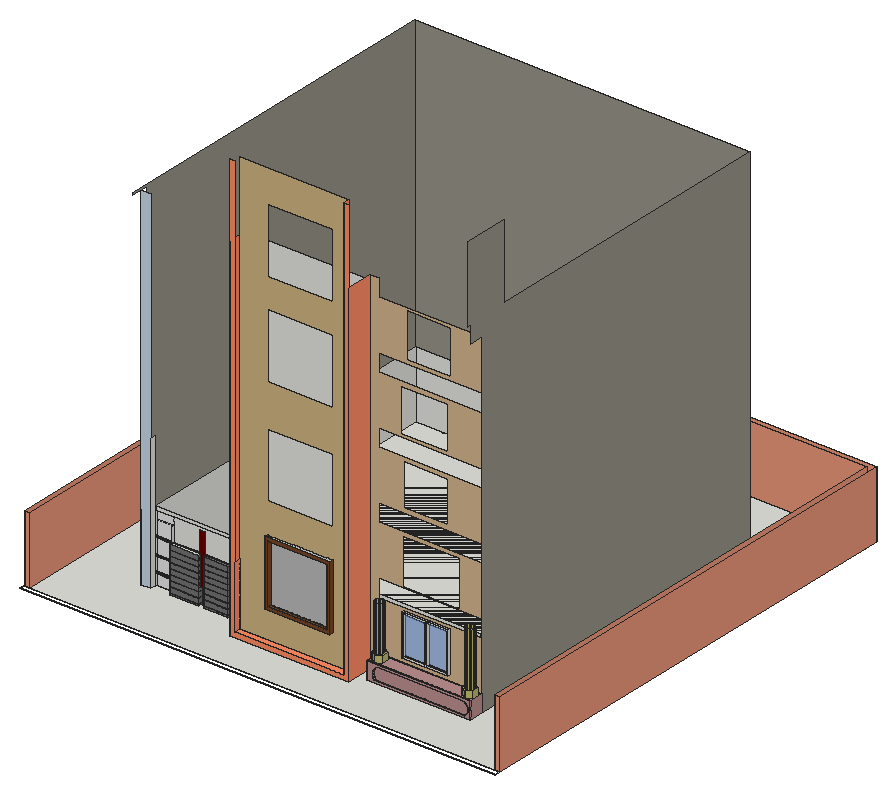
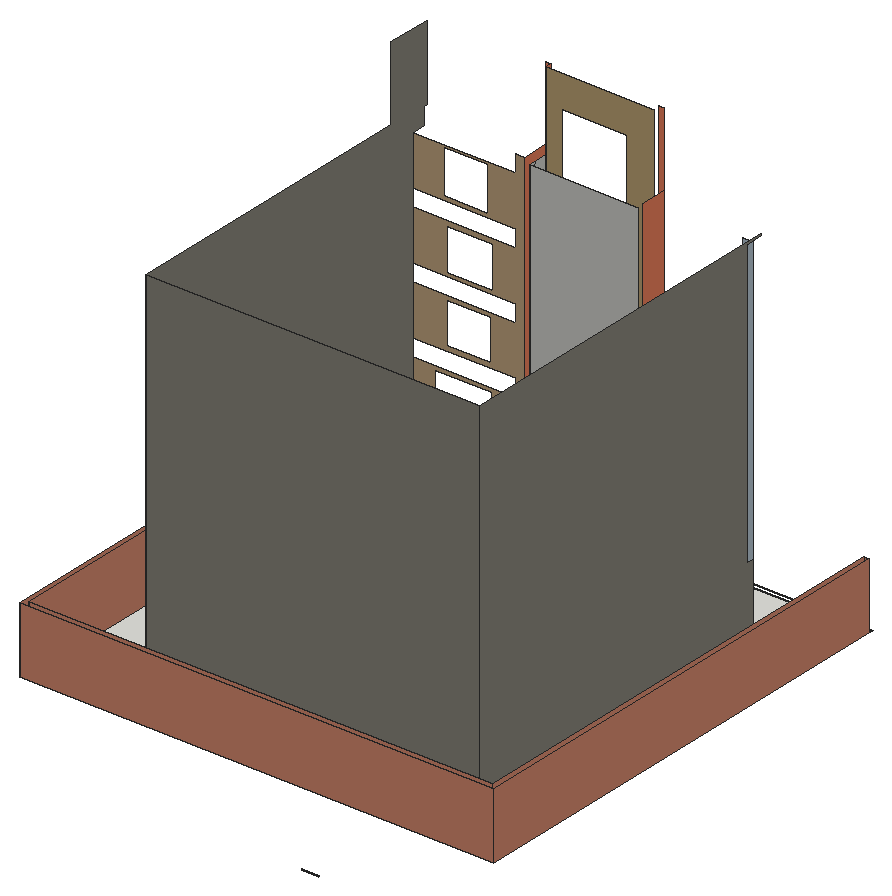
# SketchUp Ruby script. Lengths in inches.
U = 1.inch
M = Sketchup.active_model
def pt(a) = Geom::Point3d.new(a.map { |v| v * U })
def face(e, loops, mat)
  f = e.add_face(loops[0].map { |a| pt(a) })
  loops[1..].each { |l| e.add_face(l.map { |a| pt(a) }).erase! }
  f.material = f.back_material = mat if mat
  f
end
# faces: each face lists its corners as indices into pts; further lists are holes
def faces(e, pts, list, mat = nil) = list.each { |f| face(e, (f[0].is_a?(Array) ? f : [f]).map { |l| l.map { |i| pts[i] } }, mat) }
# xy, xz, yz: faces in a plane at the given z, y or x. An outline is a flat list of corners, or four numbers for a rectangle; further outlines are holes
def ring(l) = l.size == 4 ? [[l[0], l[1]], [l[2], l[1]], [l[2], l[3]], [l[0], l[3]]] : l.each_slice(2).to_a
def flat(e, list, mat, &to3) = list.each { |f| face(e, (f[0].is_a?(Array) ? f : [f]).map { |l| ring(l).map { |u, v| to3.(u, v) } }, mat) }
def xy(e, z, list, mat = nil) = flat(e, list, mat) { |x, y| [x, y, z] }
def xz(e, y, list, mat = nil) = flat(e, list, mat) { |x, z| [x, y, z] }
def yz(e, x, list, mat = nil) = flat(e, list, mat) { |y, z| [x, y, z] }
def lines(e, pts, list) = list.each { |a, b| e.add_line(pt(pts[a]), pt(pts[b])) }
# prism: a flat outline (further loops are holes) pulled along v
def prism(e, loops, v, mat = nil)
  f = face(e, loops, mat); d = Geom::Vector3d.new(v.map { |x| x * U })
  f.pushpull(f.normal.samedirection?(d) ? d.length : -d.length)
end
def box(e, o, s, mat = nil) = prism(e, [[o, [o[0] + s[0], o[1], o[2]], [o[0] + s[0], o[1] + s[1], o[2]], [o[0], o[1] + s[1], o[2]]]], [0, 0, s[2]], mat)
def at(x, y, z, deg = 0) = Geom::Transformation.translation(pt([x, y, z])) * Geom::Transformation.rotation(ORIGIN, Z_AXIS, deg.degrees)
def axes(o, x, y, z) = Geom::Transformation.new([*x, 0, *y, 0, *z, 0, *pt(o).to_a, 1])
def part(name) = M.definitions.add(name)
# library, detail: a bought-in or finely detailed component or shape, given as its bounding box
def library(name, o, s) = part(name).tap { |d| box(d.entities, o, s) }
def detail(e, o, s) = box(e.add_group.entities, o, s)
def put(e, d, t, mat = nil) = e.add_instance(d, t).tap { |i| i.material = mat if mat }
def group(e, t, mat = nil) = e.add_group.tap { |g| g.transformation = t; g.material = mat if mat }.entities
root = M.entities
M.materials.add("[0014_DarkSalmon]").color = [233, 150, 122]
M.materials.add("[0035_Tan]").color = [210, 180, 140]
M.materials.add("[0057_DarkKhaki]").color = [189, 183, 107]
M.materials.add("[0119_RosyBrown]").color = [188, 143, 143]
M.materials.add("[Color A08]").color = [102, 0, 0]
M.materials.add("[Color B03]").color = [255, 140, 101]
M.materials.add("[Color M05]").color = [114, 114, 114]
M.materials.add("[Color M09]").color = [0, 0, 0]
M.materials.add("[Formica Graystone]").color = [149, 146, 135]
M.materials.add("[Mirror 01]").color = [185, 185, 185]
M.materials.add("[Mirror 02]").color = [229, 229, 229]
M.materials.add("[Stone Sandstone Ashlar Light]").color = [206, 178, 128]
M.materials.add("[Terrazzo Light Blue]").color = [196, 214, 227]
M.materials.add("[Translucent Glass Blue]").color = [100, 149, 237]
M.materials["[Translucent Glass Blue]"].alpha = 0.5
M.materials.add("[Wood Veneer 01]").color = [120, 70, 37]
xy(root,0,[[0,0,0,841.73,850.73,841.73,850.73,0,841.73,0,841.73,832.73,9,832.73,9,0],[[9,0,841.73,832.73],[312.71,68.37,525.05,104.37],[540.59,89.37,725.37,92.37],[173.97,107.37,226.48,113.37],[235.11,107.37,278.99,113.37],[309.83,113.37,312.71,116.37],[142.36,113.37,143.68,116.37]],[[312.71,68.37,312.71,113.37,309.83,113.37,309.83,116.37,278.99,116.37,278.99,107.37,235.11,107.37,235.11,113.37,226.48,113.37,226.48,107.37,173.97,107.37,173.97,116.37,143.68,116.37,143.68,113.37,142.36,113.37,142.36,104.37,125.37,104.37,125.37,716.37,725.37,716.37,725.37,89.37,540.59,89.37,540.59,116.37,525.05,116.37,525.05,68.37],[0,-9,850.73,0]],[312.71,68.37,525.05,104.37],[540.59,89.37,725.37,92.37],
  [540.59,92.37,725.37,116.37],[[125.37,104.37,125.37,716.37,725.37,716.37,725.37,116.37,525.05,116.37,525.05,104.37,312.71,104.37,312.71,116.37,142.36,116.37,142.36,104.37],[134.37,125.37,716.37,707.37]],[173.97,107.37,183.17,113.37],[183.17,107.37,226.48,113.37],[235.11,107.37,278.99,113.37],
  [142.36,113.37,143.68,116.37],[173.97,113.37,278.99,116.37],[309.83,113.37,312.71,116.37],[134.37,125.37,716.37,707.37]])
xy(root,2.25,[[173.97,107.37,226.48,113.37]])
xy(root,3,[[555.14,89.37,714.79,92.37]],"[0119_RosyBrown]")
xy(root,3,[[235.11,107.37,278.99,113.37]],"[Color M05]")
xy(root,3.25,[[173.97,107.37,183.17,113.37],[183.17,107.37,226.48,113.37]])
xy(root,3.9375,[[235.11,107.37,278.99,113.37]])
xy(root,9,[[321.71,80.37,516.05,104.37],[321.71,104.37,516.05,116.37]])
xy(root,9,[[321.71,68.37,516.05,80.37]],"[Color B03]")
xy(root,12.0625,[[173.97,107.37,226.48,113.37]])
xy(root,12.75,[[235.11,107.37,278.99,113.37]],"[Color M05]")
xy(root,13.0625,[[173.97,107.37,183.17,113.37],[183.17,107.37,226.48,113.37]])
xy(root,13.6875,[[235.11,107.37,278.99,113.37]])
xy(root,21.05,[[143.99,113.37,173.97,116.37],[278.99,113.37,309.83,116.37]],"[Color M09]")
xy(root,21.875,[[173.97,107.37,226.48,113.37]])
xy(root,22.5,[[235.11,107.37,278.99,113.37]],"[Color M05]")
xy(root,22.62,[[143.99,113.37,173.97,116.37],[278.99,113.37,309.83,116.37]],"[Color M09]")
xy(root,22.875,[[173.97,107.37,183.17,113.37],[183.17,107.37,226.48,113.37]])
xy(root,23.4375,[[235.11,107.37,278.99,113.37]])
xy(root,27.5,[[560.89,89.37,711.42,92.37]],"[0119_RosyBrown]")
xy(root,28.6875,[[226.48,110.37,235.11,113.37]],"[Color A08]")
xy(root,30.5,[[714.82,92.2,715.1,92.37,714.53,92.37]])
xy(root,30.5,[[540.59,89.37,725.37,89.37,725.37,92.37,715.1,92.37,714.82,92.2,714.53,92.37,540.59,92.37],[540.59,92.37,552.4,92.37,543,97.8,543,108.98,552.69,114.58,562.38,108.98,562.38,97.8,552.98,92.37,714.53,92.37,705.13,97.8,705.13,108.98,714.82,114.58,724.5,108.98,724.5,97.8,715.1,92.37,725.37,92.37,725.37,116.37,540.59,116.37]],"[0119_RosyBrown]")
xy(root,31.6875,[[173.97,107.37,226.48,113.37]])
xy(root,32.25,[[235.11,107.37,278.99,113.37]],"[Color M05]")
xy(root,32.6875,[[173.97,107.37,183.17,113.37],[183.17,107.37,226.48,113.37]])
xy(root,33.1875,[[235.11,107.37,278.99,113.37]])
xy(root,39.82,[[585.01,113.37,667.64,116.37]])
xy(root,41.5,[[173.97,107.37,226.48,113.37]])
xy(root,42,[[235.11,107.37,278.99,113.37]],"[Color M05]")
xy(root,42.5,[[173.97,107.37,183.17,113.37],[183.17,107.37,226.48,113.37]])
xy(root,42.5,[[[552.4,92.37,552.98,92.37,562.38,97.8,562.38,108.98,552.69,114.58,543,108.98,543,97.8],[551.85,96.57,549.98,96.8125,548.23,97.54,546.72,98.69,545.57,100.19,544.85,101.94,544.6,103.82,544.85,105.69,545.57,107.44,546.72,108.94,548.23,110.1,549.98,110.82,551.85,111.07,553.73,110.82,555.48,110.1,556.98,108.94,558.13,107.44,558.85,105.69,559.1,103.82,558.85,101.94,558.13,100.19,556.98,98.69,555.48,97.54,553.73,96.8125]],[[714.53,92.37,715.1,92.37,724.5,97.8,724.5,108.98,714.82,114.58,705.13,108.98,705.13,97.8],[714.79,96.57,712.91,96.8125,711.16,97.54,709.66,98.69,708.51,100.19,707.79,101.94,707.54,103.82,707.79,105.69,708.51,107.44,709.66,108.94,711.16,110.1,712.91,110.82,714.79,111.07,716.67,110.82,718.41,110.1,719.92,108.94,721.07,107.44,721.79,105.69,722.04,103.82,721.79,101.94,721.07,100.19,719.92,98.69,718.41,97.54,716.67,96.8125]]],"[0057_DarkKhaki]")
xy(root,42.82,[[588.01,113.37,626.32,116.37],[629.68,113.37,664.64,116.37]])
xy(root,42.9375,[[235.11,107.37,278.99,113.37]])
xy(root,47.92,[[278.99,113.37,309.83,116.37]],"[Color M09]")
xy(root,48.86,[[143.99,113.37,173.97,116.37]],"[Color M09]")
xy(root,49.5,[[278.99,113.37,309.83,116.37]],"[Color M09]")
xy(root,50.43,[[143.99,113.37,173.97,116.37]],"[Color M09]")
xy(root,51.3125,[[173.97,107.37,226.48,113.37]])
xy(root,51.75,[[235.11,107.37,278.99,113.37]],"[Color M05]")
xy(root,52.3125,[[173.97,107.37,183.17,113.37],[183.17,107.37,226.48,113.37]])
xy(root,52.6875,[[235.11,107.37,278.99,113.37]])
xy(root,60.06,[[370.4,74.37,487.09,80.37]],"[Wood Veneer 01]")
xy(root,61.125,[[173.97,107.37,226.48,113.37]])
xy(root,61.5,[[235.11,107.37,278.99,113.37]],"[Color M05]")
xy(root,62.125,[[173.97,107.37,183.17,113.37],[183.17,107.37,226.48,113.37]])
xy(root,62.4375,[[235.11,107.37,278.99,113.37]])
xy(root,66.06,[[376.4,74.37,481.09,80.37]],"[Wood Veneer 01]")
xy(root,70.9375,[[173.97,107.37,226.48,113.37]])
xy(root,71.25,[[235.11,107.37,278.99,113.37]],"[Color M05]")
xy(root,71.9375,[[173.97,107.37,183.17,113.37],[183.17,107.37,226.48,113.37]])
xy(root,72.1875,[[235.11,107.37,278.99,113.37]])
xy(root,76.3,[[278.99,113.37,309.83,116.37]],"[Color M09]")
xy(root,77.87,[[278.99,113.37,309.83,116.37]],"[Color M09]")
xy(root,78.98,[[143.99,113.37,173.97,116.37]],"[Color M09]")
xy(root,80.56,[[143.99,113.37,173.97,116.37]],"[Color M09]")
xy(root,80.75,[[173.97,107.37,226.48,113.37]])
xy(root,81,[[235.11,107.37,278.99,113.37]],"[Color M05]")
xz(root,0,[[0,0,9,120],[841.73,0,850.73,120]],"[0014_DarkSalmon]")
xz(root,68.37,[[312.71,0,525.05,0,525.05,764.5625,516.05,764.5625,516.05,9,321.71,9,321.71,764.5625,312.71,764.5625]],"[Color B03]")
xz(root,74.37,[[[370.4,60.06,487.09,176.74],[376.4,66.06,481.09,170.74]]],"[Wood Veneer 01]")
xz(root,80.37,[[[370.4,60.06,487.09,176.74],[376.4,66.06,481.09,170.74]]])
xz(root,80.37,[[376.4,66.06,481.09,170.74]],"[Mirror 01]")
xz(root,80.37,[[[321.71,9,516.05,764.5625],[370.4,590.49,487.09,707.18],[370.4,421.56,487.09,538.24],[370.4,230.12,487.09,346.81],[370.4,60.06,487.09,176.74]]],"[Stone Sandstone Ashlar Light]")
xz(root,89.37,[[[540.59,0,725.37,30.5],[555.14,3,553.76,4.99,552.69,7.16,551.97,9.47,551.61,11.86,551.62,14.27,551.99,16.66,552.72,18.97,553.79,21.14,555.18,23.12,556.85,24.86,558.77,26.34,560.89,27.5,711.42,27.5,713.98,26.7,716.33,25.38,718.36,23.62,719.99,21.48,721.15,19.06,721.78,16.45,721.875,13.76,721.42,11.11,720.43,8.61,718.95,6.37,717.05,4.47,714.79,3]]],"[0119_RosyBrown]")
xz(root,92.37,[[[540.59,0,725.37,30.5],[555.14,3,714.79,3,717.05,4.47,718.95,6.37,720.43,8.61,721.42,11.11,721.875,13.76,721.78,16.45,721.15,19.06,719.99,21.48,718.36,23.62,716.33,25.38,713.98,26.7,711.42,27.5,560.89,27.5,558.77,26.34,556.85,24.86,555.18,23.12,553.79,21.14,552.72,18.97,551.99,16.66,551.62,14.27,551.61,11.86,551.97,9.47,552.69,7.16,553.76,4.99]],[552.4,30.5,552.98,42.5]])
xz(root,92.37,[[714.53,30.5,715.1,42.5]],"[0057_DarkKhaki]")
xz(root,92.37,[[555.14,3,714.79,3,717.05,4.47,718.95,6.37,720.43,8.61,721.42,11.11,721.875,13.76,721.78,16.45,721.15,19.06,719.99,21.48,718.36,23.62,716.33,25.38,713.98,26.7,711.42,27.5,560.89,27.5,558.77,26.34,556.85,24.86,555.18,23.12,553.79,21.14,552.72,18.97,551.99,16.66,551.62,14.27,551.61,11.86,551.97,9.47,552.69,7.16,553.76,4.99]],"[0119_RosyBrown]")
xz(root,104.37,[[125.37,0,142.36,632]],"[Terrazzo Light Blue]")
xz(root,107.37,[[173.97,0,226.48,2.25],[235.11,0,278.99,3],[173.97,3.25,226.48,12.0625],[235.11,3.9375,278.99,12.75],[173.97,13.0625,226.48,21.875],
  [235.11,13.6875,278.99,22.5],[173.97,22.875,226.48,31.6875],[235.11,23.4375,278.99,32.25],[173.97,32.6875,226.48,41.5],[235.11,33.1875,278.99,42],
  [173.97,42.5,226.48,51.3125],[235.11,42.9375,278.99,51.75],[173.97,52.3125,226.48,61.125],[235.11,52.6875,278.99,61.5],[173.97,62.125,226.48,70.9375],
  [235.11,62.4375,278.99,71.25],[173.97,71.9375,226.48,80.75],[235.11,72.1875,278.99,81]],"[Color M05]")
xz(root,110.37,[[226.48,28.6875,235.11,120]],"[Color A08]")
xz(root,113.37,[[142.36,0,143.68,120],[173.97,0,183.17,2.25],[227.05,0,235.11,0,235.11,3,278.99,3,278.99,3.9375,235.11,3.9375,235.11,12.75,278.99,12.75,278.99,13.6875,235.11,13.6875,235.11,22.5,278.99,22.5,278.99,23.4375,235.11,23.4375,235.11,28.6875,227.05,28.6875,227.05,22.875,173.97,22.875,173.97,21.875,227.05,21.875,227.05,13.0625,173.97,13.0625,173.97,12.0625,227.05,12.0625,227.05,3.25,173.97,3.25,173.97,2.25,227.05,2.25],[183.17,0,226.48,2.25],[235.11,0,278.99,3],
  [173.97,3.25,183.17,12.0625],[183.17,3.25,226.48,12.0625],[235.11,3.9375,278.99,12.75],[173.97,13.0625,183.17,21.875],[183.17,13.0625,226.48,21.875],
  [235.11,13.6875,278.99,22.5],[173.97,22.875,183.17,31.6875],[183.17,22.875,226.48,31.6875],[226.48,22.875,227.05,28.6875],[235.11,23.4375,278.99,32.25],
  [173.97,31.6875,226.48,32.6875],[235.11,32.25,278.99,33.1875],[173.97,32.6875,183.17,41.5],[183.17,32.6875,226.48,41.5],[235.11,33.1875,278.99,42],
  [[585.01,39.82,667.64,114.39],[588.01,42.82,626.32,111.39],[629.68,42.82,664.64,111.39]],[173.97,41.5,226.48,42.5],[235.11,42,278.99,42.9375],[173.97,42.5,183.17,51.3125],[183.17,42.5,226.48,51.3125],
  [235.11,42.9375,278.99,51.75],[173.97,51.3125,226.48,52.3125],[235.11,51.75,278.99,52.6875],[173.97,52.3125,183.17,61.125],[183.17,52.3125,226.48,61.125],
  [235.11,52.6875,278.99,61.5],[173.97,61.125,226.48,62.125],[235.11,61.5,278.99,62.4375],[173.97,62.125,183.17,70.9375],[183.17,62.125,226.48,70.9375],
  [235.11,62.4375,278.99,71.25],[173.97,70.9375,226.48,71.9375],[235.11,71.25,278.99,72.1875],[173.97,71.9375,183.17,80.75],[183.17,71.9375,226.48,80.75],
  [235.11,72.1875,278.99,81],[173.97,80.75,226.48,81.75],[235.11,81,278.99,81.9375]])
xz(root,113.37,[[226.48,0,227.05,2.25],[226.48,3.25,227.05,12.0625],[226.48,13.0625,227.05,21.875]],"[Color M05]")
xz(root,113.37,[[309.83,0,312.71,120],[143.99,21.05,173.97,22.62],[278.99,21.05,309.83,22.62],[278.99,47.92,309.83,49.5],[143.99,48.86,173.97,50.43],
  [278.99,76.3,309.83,77.87],[143.99,78.98,173.97,80.56]],"[Color M09]")
xz(root,116.37,[[540.59,-0.25,725.37,0],[142.36,0,143.68,120],[173.97,0,174.52,21.05],[174.52,0,174.52,21.05,174.83,21.05,174.83,22.62,174.52,22.62,174.52,48.86,174.83,48.86,174.83,50.43,174.52,50.43,174.52,78.98,174.83,78.98,174.83,80.56,174.52,80.56,174.52,105.17,174.83,105.17,174.83,106.75,174.52,106.75,174.52,120,278.99,120,278.99,0],[309.83,0,312.71,120],
  [540.59,0,725.37,30.5],[321.71,9,516.05,623],[143.99,21.05,173.97,22.62],[173.97,21.05,174.52,22.62],[174.52,21.05,174.83,22.62],
  [278.99,21.05,309.83,22.62],[173.97,22.62,174.52,48.86],[[585.01,39.82,667.64,114.39],[588.01,42.82,626.32,111.39],[629.68,42.82,664.64,111.39]],[278.99,47.92,309.83,49.5],[143.99,48.86,173.97,50.43],
  [173.97,48.86,174.52,50.43],[174.52,48.86,174.83,50.43],[173.97,50.43,174.52,78.98],[278.99,76.3,309.83,77.87],[143.99,78.98,173.97,80.56],
  [173.97,78.98,174.52,80.56],[174.52,78.98,174.83,80.56],[173.97,80.56,174.52,105.17]])
xz(root,116.37,[[[525.05,0,540.59,0,540.59,150.75,725.37,150.75,725.37,240.5,540.59,240.5,540.59,271.25,725.37,271.25,725.37,361,540.59,361,540.59,391.75,725.37,391.75,725.37,481.5,540.59,481.5,540.59,512.25,725.37,512.25,725.37,602,540.59,602,540.59,632,525.05,632],[583.77,151.69,686.39,234.13],[590.68,518.48,670.37,598.17],[581.28,397.08,664.4,473.26],[586.09,279.75,664.21,354.13]],[[540.59,30.5,725.37,120],[585.01,39.82,667.64,114.39]]],"[0035_Tan]")
xz(root,116.37,[[143.68,0,173.97,0,173.97,21.05,143.99,21.05,143.99,22.62,173.97,22.62,173.97,48.86,143.99,48.86,143.99,50.43,173.97,50.43,173.97,78.98,143.99,78.98,143.99,80.56,173.97,80.56,173.97,105.17,143.99,105.17,143.99,106.75,173.97,106.75,173.97,120,143.68,120],[278.99,0,309.83,21.05],[278.99,22.62,309.83,47.92],[278.99,49.5,309.83,76.3],[278.99,77.87,309.83,101.48]],"[Mirror 02]")
xz(root,116.37,[[588.01,42.82,626.32,111.39],[629.68,42.82,664.64,111.39]],"[Translucent Glass Blue]")
xz(root,125.37,[[134.37,0,716.37,120]])
xz(root,707.37,[[134.37,0,716.37,120]])
xz(root,716.37,[[125.37,0,725.37,636]],"[Formica Graystone]")
xz(root,832.73,[[9,0,841.73,120]],"[0014_DarkSalmon]")
xz(root,841.73,[[0,0,850.73,120]],"[0014_DarkSalmon]")
xz(root,1053.87,[[143.99,21.05,173.97,22.62]])
yz(root,0,[[0,0,841.73,120]],"[0014_DarkSalmon]")
yz(root,9,[[0,0,832.73,120]],"[0014_DarkSalmon]")
yz(root,125.37,[[104.37,0,104.37,120,116.37,120,116.37,632,85.68,632,85.68,636,716.37,636,716.37,0]],"[Formica Graystone]")
yz(root,134.37,[[125.37,0,707.37,120]])
yz(root,142.36,[[104.37,0,113.37,240],[113.37,0,116.37,120]])
yz(root,143.68,[[113.37,0,116.37,120]])
yz(root,143.99,[[113.37,21.05,116.37,22.62],[113.37,48.86,116.37,50.43],[113.37,78.98,116.37,80.56]])
yz(root,173.97,[[107.37,0,113.37,2.25],[113.37,0,116.37,21.05],[113.37,21.05,116.37,22.62],[113.37,22.62,116.37,48.86],[113.37,48.86,116.37,50.43],
  [113.37,50.43,116.37,78.98],[113.37,78.98,116.37,80.56],[113.37,80.56,116.37,105.17]])
yz(root,173.97,[[107.37,3.25,113.37,12.0625],[107.37,13.0625,113.37,21.875],[107.37,22.875,113.37,31.6875],[107.37,32.6875,113.37,41.5],[107.37,42.5,113.37,51.3125],
  [107.37,52.3125,113.37,61.125],[107.37,62.125,113.37,70.9375],[107.37,71.9375,113.37,80.75]],"[Color M05]")
yz(root,226.48,[[110.37,28.6875,113.37,31.6875],[110.37,31.6875,113.37,32.6875],[110.37,32.6875,113.37,41.5],[110.37,41.5,113.37,42.5],[110.37,42.5,113.37,51.3125],
  [110.37,51.3125,113.37,52.3125],[110.37,52.3125,113.37,61.125],[110.37,61.125,113.37,62.125],[110.37,62.125,113.37,70.9375],[110.37,70.9375,113.37,71.9375],
  [110.37,71.9375,113.37,80.75],[110.37,80.75,113.37,81.75]])
yz(root,226.48,[[107.37,0,113.37,2.25],[107.37,3.25,113.37,12.0625],[107.37,13.0625,113.37,21.875],[107.37,22.875,113.37,28.6875],[107.37,28.6875,110.37,31.6875],
  [107.37,32.6875,110.37,41.5],[107.37,42.5,110.37,51.3125],[107.37,52.3125,110.37,61.125],[107.37,62.125,110.37,70.9375],[107.37,71.9375,110.37,80.75]],"[Color M05]")
yz(root,235.11,[[110.37,28.6875,113.37,32.25],[110.37,32.25,113.37,33.1875],[110.37,33.1875,113.37,42],[110.37,42,113.37,42.9375],[110.37,42.9375,113.37,51.75],
  [110.37,51.75,113.37,52.6875],[110.37,52.6875,113.37,61.5],[110.37,61.5,113.37,62.4375],[110.37,62.4375,113.37,71.25],[110.37,71.25,113.37,72.1875],
  [110.37,72.1875,113.37,81],[110.37,81,113.37,81.9375]])
yz(root,235.11,[[107.37,0,113.37,3],[107.37,3.9375,113.37,12.75],[107.37,13.6875,113.37,22.5],[107.37,23.4375,113.37,28.6875],[107.37,28.6875,110.37,32.25],
  [107.37,33.1875,110.37,42],[107.37,42.9375,110.37,51.75],[107.37,52.6875,110.37,61.5],[107.37,62.4375,110.37,71.25],[107.37,72.1875,110.37,81]],"[Color M05]")
yz(root,278.99,[[113.37,21.05,116.37,22.62],[113.37,47.92,116.37,49.5],[113.37,76.3,116.37,77.87]])
yz(root,278.99,[[107.37,0,113.37,3],[113.37,0,116.37,21.05],[107.37,3.9375,113.37,12.75],[107.37,13.6875,113.37,22.5],[113.37,22.62,116.37,47.92],
  [107.37,23.4375,113.37,32.25],[107.37,33.1875,113.37,42],[107.37,42.9375,113.37,51.75],[113.37,49.5,116.37,76.3],[107.37,52.6875,113.37,61.5],
  [107.37,62.4375,113.37,71.25],[107.37,72.1875,113.37,81],[113.37,77.87,116.37,101.48]],"[Color M05]")
yz(root,309.83,[[113.37,21.05,116.37,22.62],[113.37,47.92,116.37,49.5],[113.37,76.3,116.37,77.87]])
yz(root,309.83,[[113.37,0,116.37,21.05],[113.37,22.62,116.37,47.92],[113.37,49.5,116.37,76.3],[113.37,77.87,116.37,101.48]],"[Color M09]")
yz(root,312.71,[[104.37,0,113.37,120],[113.37,0,116.37,120]])
yz(root,312.71,[[68.37,0,68.37,632,116.37,632,116.37,120,104.37,120,104.37,0]],"[Color B03]")
yz(root,321.71,[[80.37,9,104.37,120],[104.37,9,116.37,120]])
yz(root,321.71,[[68.37,9,80.37,120]],"[Color B03]")
yz(root,370.4,[[74.37,60.06,80.37,176.74]],"[Wood Veneer 01]")
yz(root,376.4,[[74.37,66.06,80.37,170.74]],"[Wood Veneer 01]")
yz(root,481.09,[[74.37,66.06,80.37,170.74]],"[Wood Veneer 01]")
yz(root,487.09,[[74.37,60.06,80.37,176.74]],"[Wood Veneer 01]")
yz(root,516.05,[[80.37,9,104.37,623],[104.37,9,116.37,623]])
yz(root,516.05,[[68.37,9,80.37,764.5625]],"[Color B03]")
yz(root,525.05,[[68.37,0,116.37,632]],"[Color B03]")
yz(root,540.59,[[89.37,0,92.37,3.625]])
yz(root,540.59,[[92.37,0,116.37,3.625],[89.37,3.625,92.37,30.5],[92.37,3.625,116.37,30.5]],"[0119_RosyBrown]")
yz(root,543,[[97.8,30.5,108.98,42.5]])
yz(root,562.38,[[97.8,30.5,108.98,42.5]],"[0057_DarkKhaki]")
yz(root,585.01,[[113.37,39.82,116.37,114.39]])
yz(root,588.01,[[113.37,42.82,116.37,111.39]])
yz(root,626.32,[[113.37,42.82,116.37,111.39]])
yz(root,629.68,[[113.37,42.82,116.37,111.39]])
yz(root,664.64,[[113.37,42.82,116.37,111.39]])
yz(root,667.64,[[113.37,39.82,116.37,114.39]])
yz(root,705.13,[[97.8,30.5,108.98,42.5]],"[0057_DarkKhaki]")
yz(root,716.37,[[125.37,0,707.37,120]])
yz(root,724.5,[[97.8,30.5,108.98,42.5]],"[0057_DarkKhaki]")
yz(root,725.37,[[89.37,0,92.37,30.5],[92.37,0,116.37,30.5]],"[0119_RosyBrown]")
yz(root,725.37,[[116.37,0,716.37,0,716.37,636,165.62,636,165.62,768.6875,85.68,768.6875,85.68,632,92.37,632,92.37,602,116.37,602]],"[Formica Graystone]")
yz(root,841.73,[[0,0,832.73,120]],"[0014_DarkSalmon]")
yz(root,850.73,[[0,0,841.73,120]],"[0014_DarkSalmon]")
p = [[555.14,92.37,3],[553.76,92.37,4.99],[553.76,89.37,4.99],[555.14,89.37,3],[717.05,92.37,4.47],[714.79,92.37,3],
  [714.79,89.37,3],[717.05,89.37,4.47],[718.95,92.37,6.37],[718.95,89.37,6.37],[552.69,92.37,7.16],[552.69,89.37,7.16],
  [720.43,92.37,8.61],[720.43,89.37,8.61],[551.97,92.37,9.47],[551.97,89.37,9.47],[721.42,92.37,11.11],[721.42,89.37,11.11],
  [551.61,92.37,11.86],[551.61,89.37,11.86],[721.875,92.37,13.76],[721.875,89.37,13.76],[551.62,92.37,14.27],[551.62,89.37,14.27],
  [721.78,92.37,16.45],[721.78,89.37,16.45],[551.99,92.37,16.66],[551.99,89.37,16.66],[721.15,92.37,19.06],[721.15,89.37,19.06],
  [552.72,92.37,18.97],[552.72,89.37,18.97],[553.79,92.37,21.14],[553.79,89.37,21.14],[719.99,92.37,21.48],[719.99,89.37,21.48],
  [555.18,92.37,23.12],[555.18,89.37,23.12],[718.36,92.37,23.62],[718.36,89.37,23.62],[556.85,92.37,24.86],[556.85,89.37,24.86],
  [716.33,92.37,25.38],[716.33,89.37,25.38],[558.77,92.37,26.34],[558.77,89.37,26.34],[713.98,92.37,26.7],[713.98,89.37,26.7],
  [560.89,92.37,27.5],[560.89,89.37,27.5],[711.42,92.37,27.5],[711.42,89.37,27.5],[543,97.8,30.5],[552.4,92.37,30.5],
  [552.4,92.37,42.5],[543,97.8,42.5],[552.98,92.37,30.5],[562.38,97.8,30.5],[562.38,97.8,42.5],[552.98,92.37,42.5],
  [705.13,97.8,30.5],[714.53,92.37,30.5],[714.53,92.37,42.5],[705.13,97.8,42.5],[715.1,92.37,30.5],[724.5,97.8,30.5],
  [724.5,97.8,42.5],[715.1,92.37,42.5],[552.69,114.58,30.5],[543,108.98,30.5],[543,108.98,42.5],[552.69,114.58,42.5],
  [562.38,108.98,30.5],[562.38,108.98,42.5],[714.82,114.58,30.5],[705.13,108.98,30.5],[705.13,108.98,42.5],[714.82,114.58,42.5],
  [724.5,108.98,30.5],[724.5,108.98,42.5],[549.98,96.8125,42.5],[551.85,96.57,42.5],[551.85,96.57,123.625],[549.98,96.8125,123.625],
  [553.73,96.8125,42.5],[553.73,96.8125,123.625],[712.91,96.8125,42.5],[714.79,96.57,42.5],[714.79,96.57,139.875],[712.91,96.8125,139.875],
  [716.67,96.8125,42.5],[716.67,96.8125,139.875],[548.23,97.54,42.5],[548.23,97.54,123.625],[555.48,97.54,42.5],[555.48,97.54,123.625],
  [711.16,97.54,42.5],[711.16,97.54,139.875],[718.41,97.54,42.5],[718.41,97.54,139.875],[546.72,98.69,42.5],[546.72,98.69,123.625],
  [556.98,98.69,42.5],[556.98,98.69,123.625],[709.66,98.69,42.5],[709.66,98.69,139.875],[719.92,98.69,42.5],[719.92,98.69,139.875],
  [545.57,100.19,42.5],[545.57,100.19,123.625],[558.13,100.19,42.5],[558.13,100.19,123.625],[708.51,100.19,42.5],[708.51,100.19,139.875],
  [721.07,100.19,42.5],[721.07,100.19,139.875],[544.85,101.94,42.5],[544.85,101.94,123.625],[558.85,101.94,42.5],[558.85,101.94,123.625],
  [707.79,101.94,42.5],[707.79,101.94,139.875],[721.79,101.94,42.5],[721.79,101.94,139.875],[544.6,103.82,42.5],[544.6,103.82,123.625],
  [559.1,103.82,42.5],[559.1,103.82,123.625],[707.54,103.82,42.5],[707.54,103.82,139.875],[722.04,103.82,42.5],[722.04,103.82,139.875],
  [544.85,105.69,42.5],[544.85,105.69,123.625],[558.85,105.69,42.5],[558.85,105.69,123.625],[707.79,105.69,42.5],[707.79,105.69,139.875],
  [721.79,105.69,42.5],[721.79,105.69,139.875],[545.57,107.44,42.5],[545.57,107.44,123.625],[558.13,107.44,42.5],[558.13,107.44,123.625],
  [708.51,107.44,42.5],[708.51,107.44,139.875],[721.07,107.44,42.5],[721.07,107.44,139.875],[546.72,108.94,42.5],[546.72,108.94,123.625],
  [556.98,108.94,42.5],[556.98,108.94,123.625],[709.66,108.94,42.5],[709.66,108.94,139.875],[719.92,108.94,42.5],[719.92,108.94,139.875],
  [548.23,110.1,42.5],[548.23,110.1,123.625],[555.48,110.1,42.5],[555.48,110.1,123.625],[711.16,110.1,42.5],[711.16,110.1,139.875],
  [718.41,110.1,42.5],[718.41,110.1,139.875],[549.98,110.82,42.5],[549.98,110.82,123.625],[553.73,110.82,42.5],[553.73,110.82,123.625],
  [712.91,110.82,42.5],[712.91,110.82,139.875],[716.67,110.82,42.5],[716.67,110.82,139.875],[551.85,111.07,42.5],[551.85,111.07,123.625],
  [714.79,111.07,42.5],[714.79,111.07,139.875],[226.48,113.37,80.75],[227.05,113.37,80.75],[227.05,113.37,71.9375],[226.48,113.37,71.9375],
  [226.48,113.37,70.9375],[227.05,113.37,70.9375],[227.05,113.37,62.125],[226.48,113.37,62.125],[226.48,113.37,61.125],[227.05,113.37,61.125],
  [227.05,113.37,52.3125],[226.48,113.37,52.3125],[226.48,113.37,51.3125],[227.05,113.37,51.3125],[227.05,113.37,42.5],[226.48,113.37,42.5],
  [226.48,113.37,41.5],[227.05,113.37,41.5],[227.05,113.37,32.6875],[226.48,113.37,32.6875],[226.48,113.37,31.6875],[227.05,113.37,31.6875],
  [227.05,113.37,28.6875]]
faces(root,p,[[0,1,2,3],[4,5,6,7],[8,4,7,9],[1,10,11,2],[12,8,9,13],[10,14,15,11],[16,12,13,17],[14,18,19,15],
  [20,16,17,21],[18,22,23,19],[24,20,21,25],[22,26,27,23],[28,24,25,29],[26,30,31,27],[30,32,33,31],[34,28,29,35],
  [32,36,37,33],[38,34,35,39],[36,40,41,37],[42,38,39,43],[40,44,45,41],[46,42,43,47],[44,48,49,45],[50,46,47,51]],"[0119_RosyBrown]")
faces(root,p,[[52,53,54,55],[56,57,58,59],[60,61,62,63],[64,65,66,67],[80,81,82,83],[81,84,85,82],[86,87,88,89],[87,90,91,88],
  [92,80,83,93],[84,94,95,85],[96,86,89,97],[90,98,99,91],[100,92,93,101],[94,102,103,95],[104,96,97,105],[98,106,107,99],
  [108,100,101,109],[102,110,111,103],[112,104,105,113],[106,114,115,107],[116,108,109,117],[110,118,119,111],[120,112,113,121],[114,122,123,115],
  [124,116,117,125],[118,126,127,119],[128,120,121,129],[122,130,131,123],[132,124,125,133],[126,134,135,127],[136,128,129,137],[130,138,139,131],
  [140,132,133,141],[134,142,143,135],[144,136,137,145],[138,146,147,139],[148,140,141,149],[142,150,151,143],[152,144,145,153],[146,154,155,147],
  [156,148,149,157],[150,158,159,151],[160,152,153,161],[154,162,163,155],[164,156,157,165],[158,166,167,159],[168,160,161,169],[162,170,171,163],
  [172,164,165,173],[166,172,173,167],[174,168,169,175],[170,174,175,171]],"[0057_DarkKhaki]")
faces(root,p,[[68,69,70,71],[72,68,71,73],[74,75,76,77],[78,74,77,79]])
lines(root,p,[[176,177],[178,179],[178,177],[180,181],[182,183],[182,181],[184,185],[186,187],[188,189],[190,191],[192,193],[194,195],
  [196,197],[186,185],[190,189],[194,193],[198,197]])
